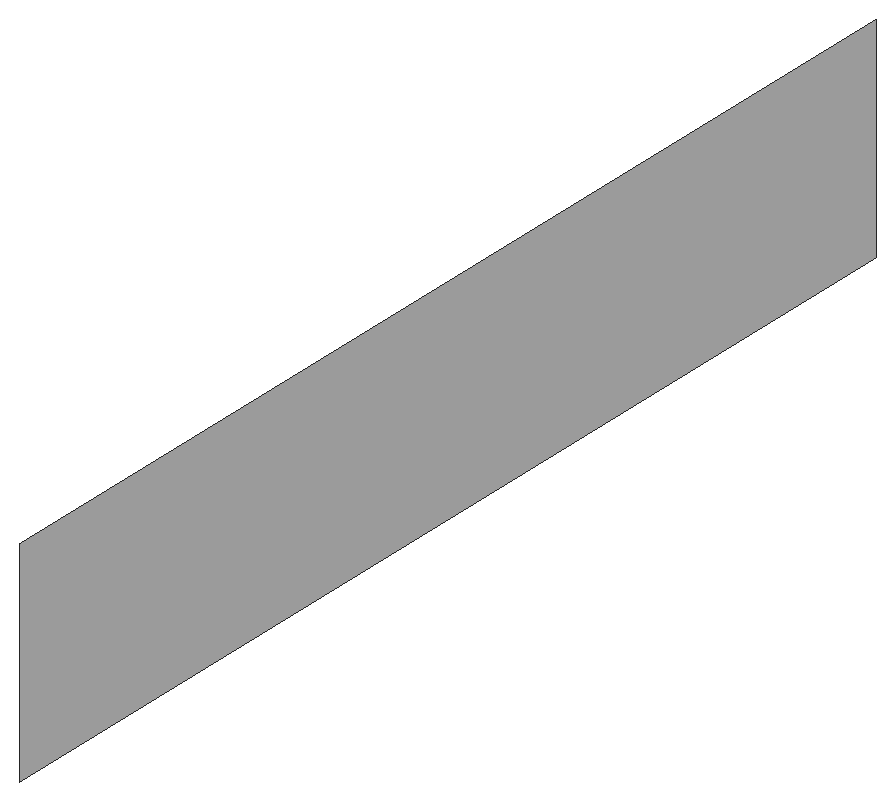
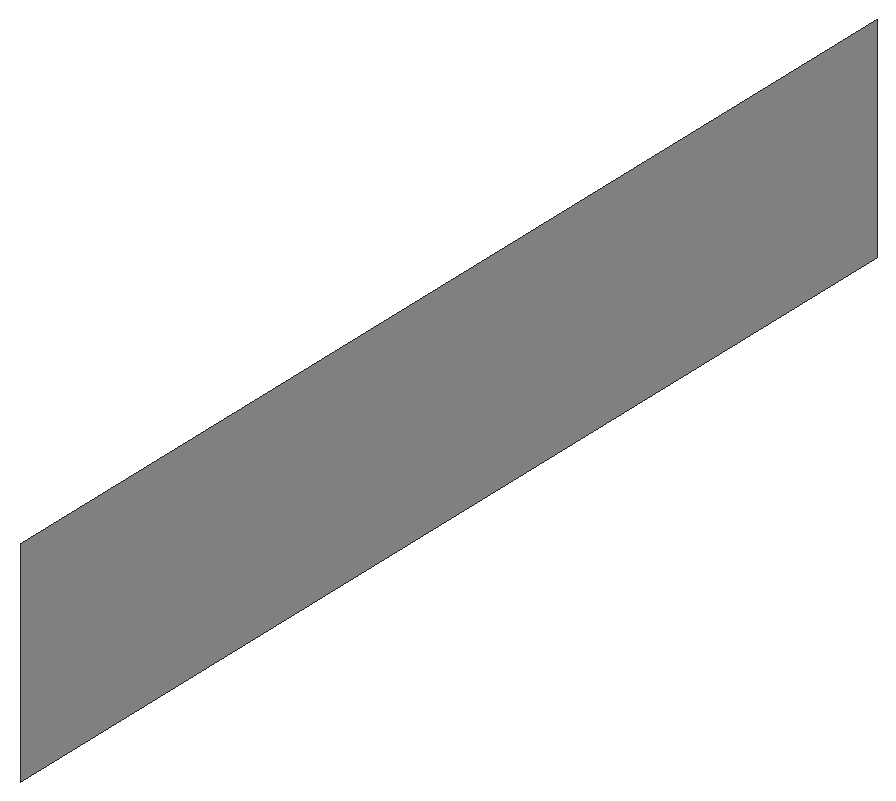
# SketchUp Ruby script. Lengths in inches.
U = 1.inch
M = Sketchup.active_model
def pt(a) = Geom::Point3d.new(a.map { |v| v * U })
def face(e, loops, mat)
  f = e.add_face(loops[0].map { |a| pt(a) })
  loops[1..].each { |l| e.add_face(l.map { |a| pt(a) }).erase! }
  f.material = f.back_material = mat if mat
  f
end
# faces: each face lists its corners as indices into pts; further lists are holes
def faces(e, pts, list, mat = nil) = list.each { |f| face(e, (f[0].is_a?(Array) ? f : [f]).map { |l| l.map { |i| pts[i] } }, mat) }
# xy, xz, yz: faces in a plane at the given z, y or x. An outline is a flat list of corners, or four numbers for a rectangle; further outlines are holes
def ring(l) = l.size == 4 ? [[l[0], l[1]], [l[2], l[1]], [l[2], l[3]], [l[0], l[3]]] : l.each_slice(2).to_a
def flat(e, list, mat, &to3) = list.each { |f| face(e, (f[0].is_a?(Array) ? f : [f]).map { |l| ring(l).map { |u, v| to3.(u, v) } }, mat) }
def xy(e, z, list, mat = nil) = flat(e, list, mat) { |x, y| [x, y, z] }
def xz(e, y, list, mat = nil) = flat(e, list, mat) { |x, z| [x, y, z] }
def yz(e, x, list, mat = nil) = flat(e, list, mat) { |y, z| [x, y, z] }
def lines(e, pts, list) = list.each { |a, b| e.add_line(pt(pts[a]), pt(pts[b])) }
# prism: a flat outline (further loops are holes) pulled along v
def prism(e, loops, v, mat = nil)
  f = face(e, loops, mat); d = Geom::Vector3d.new(v.map { |x| x * U })
  f.pushpull(f.normal.samedirection?(d) ? d.length : -d.length)
end
def box(e, o, s, mat = nil) = prism(e, [[o, [o[0] + s[0], o[1], o[2]], [o[0] + s[0], o[1] + s[1], o[2]], [o[0], o[1] + s[1], o[2]]]], [0, 0, s[2]], mat)
def at(x, y, z, deg = 0) = Geom::Transformation.translation(pt([x, y, z])) * Geom::Transformation.rotation(ORIGIN, Z_AXIS, deg.degrees)
def axes(o, x, y, z) = Geom::Transformation.new([*x, 0, *y, 0, *z, 0, *pt(o).to_a, 1])
def part(name) = M.definitions.add(name)
# library, detail: a bought-in or finely detailed component or shape, given as its bounding box
def library(name, o, s) = part(name).tap { |d| box(d.entities, o, s) }
def detail(e, o, s) = box(e.add_group.entities, o, s)
def put(e, d, t, mat = nil) = e.add_instance(d, t).tap { |i| i.material = mat if mat }
def group(e, t, mat = nil) = e.add_group.tap { |g| g.transformation = t; g.material = mat if mat }.entities
root = M.entities
M.materials.add("[Carrera Marble]").color = [207, 207, 207]
yz(root,111.93,[[162.11,70.61,233.86,84.87]],"[Carrera Marble]")
